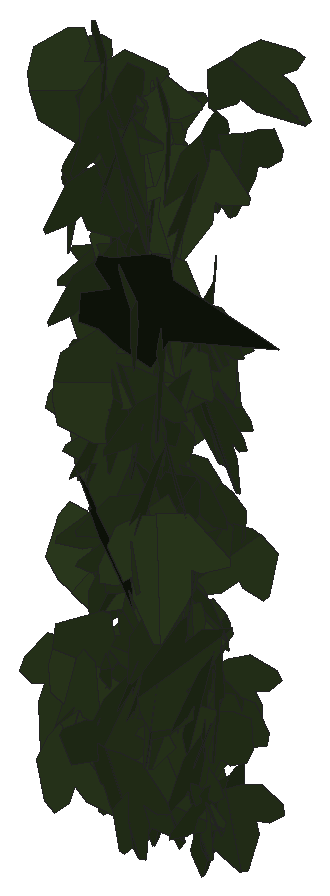
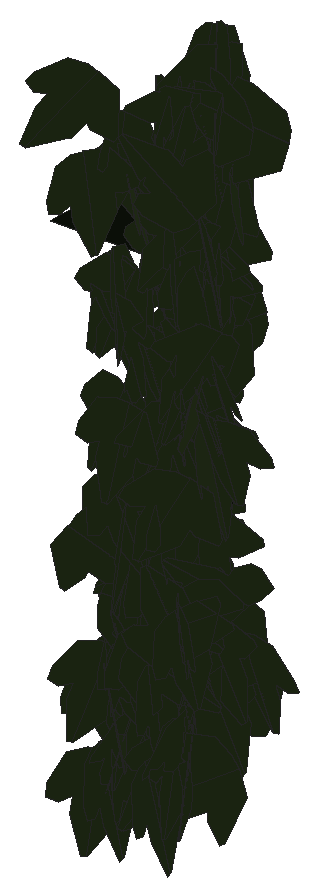
# SketchUp Ruby script. Lengths in inches.
U = 1.inch
M = Sketchup.active_model
def pt(a) = Geom::Point3d.new(a.map { |v| v * U })
def face(e, loops, mat)
  f = e.add_face(loops[0].map { |a| pt(a) })
  loops[1..].each { |l| e.add_face(l.map { |a| pt(a) }).erase! }
  f.material = f.back_material = mat if mat
  f
end
# faces: each face lists its corners as indices into pts; further lists are holes
def faces(e, pts, list, mat = nil) = list.each { |f| face(e, (f[0].is_a?(Array) ? f : [f]).map { |l| l.map { |i| pts[i] } }, mat) }
# xy, xz, yz: faces in a plane at the given z, y or x. An outline is a flat list of corners, or four numbers for a rectangle; further outlines are holes
def ring(l) = l.size == 4 ? [[l[0], l[1]], [l[2], l[1]], [l[2], l[3]], [l[0], l[3]]] : l.each_slice(2).to_a
def flat(e, list, mat, &to3) = list.each { |f| face(e, (f[0].is_a?(Array) ? f : [f]).map { |l| ring(l).map { |u, v| to3.(u, v) } }, mat) }
def xy(e, z, list, mat = nil) = flat(e, list, mat) { |x, y| [x, y, z] }
def xz(e, y, list, mat = nil) = flat(e, list, mat) { |x, z| [x, y, z] }
def yz(e, x, list, mat = nil) = flat(e, list, mat) { |y, z| [x, y, z] }
def lines(e, pts, list) = list.each { |a, b| e.add_line(pt(pts[a]), pt(pts[b])) }
# prism: a flat outline (further loops are holes) pulled along v
def prism(e, loops, v, mat = nil)
  f = face(e, loops, mat); d = Geom::Vector3d.new(v.map { |x| x * U })
  f.pushpull(f.normal.samedirection?(d) ? d.length : -d.length)
end
def box(e, o, s, mat = nil) = prism(e, [[o, [o[0] + s[0], o[1], o[2]], [o[0] + s[0], o[1] + s[1], o[2]], [o[0], o[1] + s[1], o[2]]]], [0, 0, s[2]], mat)
def at(x, y, z, deg = 0) = Geom::Transformation.translation(pt([x, y, z])) * Geom::Transformation.rotation(ORIGIN, Z_AXIS, deg.degrees)
def axes(o, x, y, z) = Geom::Transformation.new([*x, 0, *y, 0, *z, 0, *pt(o).to_a, 1])
def part(name) = M.definitions.add(name)
# library, detail: a bought-in or finely detailed component or shape, given as its bounding box
def library(name, o, s) = part(name).tap { |d| box(d.entities, o, s) }
def detail(e, o, s) = box(e.add_group.entities, o, s)
def put(e, d, t, mat = nil) = e.add_instance(d, t).tap { |i| i.material = mat if mat }
def group(e, t, mat = nil) = e.add_group.tap { |g| g.transformation = t; g.material = mat if mat }.entities
root = M.entities
M.materials.add("efeu1").color = [18, 25, 13]
M.materials.add("efeu2").color = [43, 57, 29]
c1 = part("ivyleaf_10")
p = [[0,0.5,-0.03],[-0.0625,2.02,-0.43],[-0.19,2.01,-0.46],[-0.54,1.05,-0.29],[-0.52,0.625,-0.18],[-0.83,0.76,-0.28],
  [-1.16,0.64,-0.33],[-1.15,0.33,-0.24],[-0.77,-0.39,0.02],[-0.3,-0.51,0.16],[0.04,-0.48,0.23],[-0.02,2.01,-0.4375],
  [-0.06,2.01,-0.43],[0.04,-0.49,0.23],[0.67,-0.49,0.14],[1.38,0.36,-0.2],[1.375,0.51,-0.24],[0.81,0.65,-0.19],
  [0.62,0.59,-0.15],[0.6,1.09,-0.28],[0.5,1.23,-0.31]]
faces(c1.entities,p,[[0,1,2,3,4,5,6,7,8,9,10],[11,12,0,13,14,15,16,17,18,19,20]],"efeu2")
c2 = part("ivyleaf_9")
p = [[1.54,2.16,1.25],[1.36,2.04,1.19],[-0.21,0.99,0.68],[-0.71,1.11,0.82],[-0.85,0.86,0.67],[-0.8,0.17,0.21],
  [-0.9,-0.01,0.1],[-0.67,-0.16,-0.02],[-0.08,-0.08,-0.05],[-0.03,-0.6,-0.4],[0.65,-0.88,-0.66],[0.83,-0.6,-0.49],
  [1.29,-0.42,-0.43],[1.8125,-0.07,-0.26],[1.21,0.44,0.15]]
faces(c2.entities,p,[[0,1,2,3,4,5,6,7,8,9,10,11,12,13,14]],"efeu1")
put(root,c1,axes([509.14,138.66,175.01],[-0.12487,-0.54148,0.08377],[0.01315,-0.08485,-0.57503],[0.59109,-0.1125,0.03049]))
put(root,c1,axes([509.08,137.85,177.79],[0.63301,0.02051,-0.00556],[-0.00502,-0.0199,-0.60959],[-0.02233,0.5858,-0.02052]))
put(root,c1,axes([509.17,137.07,174.02],[0.64268,-0.19201,-0.04798],[-0.04531,0.02022,-0.65026],[0.2084,0.59652,0.0066]))
put(root,c1,axes([508.87,138.21,172.65],[-0.3827,0.09507,-0.52218],[0.51482,-0.09013,-0.39371],[-0.12913,-0.6411,-0.02209]))
put(root,c1,axes([508.7,137.42,182.46],[0.14471,0.01205,-0.68867],[0.68877,-0.00317,0.14467],[-0.00062,-0.7037,-0.01244]))
put(root,c1,axes([509,137.7,175.15],[0.43863,0.21179,-0.47557],[0.31682,0.38486,0.46361],[0.4131,-0.52005,0.14941]))
put(root,c1,axes([509.18,138.58,175.14],[0.39654,-0.42737,0.03226],[0.11124,0.04837,-0.5748],[0.4492,0.36529,0.11386]))
put(root,c1,axes([509.33,138.37,175.4],[-0.35479,-0.44656,0.0359],[0.02472,-0.05949,-0.57386],[0.4831,-0.32492,0.05573]))
put(root,c1,axes([509.38,137.8,180.74],[0.31056,-0.44996,-0.20666],[-0.10102,0.17596,-0.55514],[0.52155,0.30202,0.01553]))
put(root,c1,axes([509.125,137.42,181.51],[0.19807,-0.40948,0.38674],[0.27262,-0.28664,-0.45774],[0.53156,0.29959,0.09065]))
put(root,c1,axes([509.36,138.09,172.95],[0.24083,-0.49273,-0.37457],[-0.01972,0.39561,-0.53309],[0.61862,0.20443,0.12882]))
put(root,c1,axes([509.21,138.66,174.84],[-0.26372,-0.48177,0.15292],[0.07732,0.12856,0.5617],[-0.53849,0.2544,0.00576]))
put(root,c1,axes([509.37,137.71,177.49],[0.1664,-0.66597,-0.03146],[0.00048,0.03254,-0.68639],[0.66671,0.16619,0.00834]))
put(root,c1,axes([509.41,137.53,173.38],[-0.00057,-0.57318,0.15265],[0.00419,-0.14678,-0.59609],[0.63899,0.00045,0.00404]))
put(root,c1,axes([509.5,138.43,175.24],[-0.13521,-0.39389,0.39525],[-0.05313,-0.38018,-0.42665],[0.58874,-0.12477,0.05227]))
put(root,c1,axes([509.72,137.3125,174.05],[-0.47414,-0.04836,0.35073],[-0.35876,-0.06142,-0.45889],[0.08172,-0.55018,0.0204]))
put(root,c1,axes([509.33,137.68,178.71],[0.49544,-0.37884,0.12538],[0.09205,-0.08609,-0.61862],[0.41938,0.46644,-0.01234]))
put(root,c1,axes([509.54,137.85,176.01],[-0.36134,-0.54866,0.07499],[-0.02503,-0.07327,-0.65667],[0.55319,-0.36169,0.01927]))
put(root,c1,axes([509.29,138.56,177.05],[-0.51196,-0.19796,-0.24826],[0.27307,0.00575,-0.52714],[0.19392,-0.53072,0.08689]))
put(root,c1,axes([509.29,137.89,179.07],[0.15858,0.4507,0.35105],[0.06475,0.33434,-0.4914],[-0.60468,0.154,0.03945]))
put(root,c1,axes([509.49,137.35,181.26],[-0.61777,0.06757,-0.01879],[0.02137,0.01354,-0.5988],[-0.07245,-0.57214,-0.01639]))
put(root,c1,axes([509.01,137.65,182.65],[0.00822,0.00838,-0.58657],[0.53618,-0.26787,0.00282],[-0.2892,-0.4964,-0.01143]))
put(root,c1,axes([509.39,138.36,173.36],[-0.08192,0.61733,-0.17364],[0.00439,-0.17451,-0.62249],[-0.64127,-0.08005,0.01792]))
put(root,c1,axes([509.56,137.66,179.85],[-0.08392,-0.55093,0.08387],[-0.02496,-0.07817,-0.57851],[0.60083,-0.0802,-0.01232]))
put(root,c1,axes([509.4375,137.84,178.22],[0.41126,-0.44506,0.10504],[0.06153,-0.08416,-0.60905],[0.48903,0.38487,-0.01171]))
put(root,c1,axes([509.51,138.25,176.6],[-0.11415,-0.55749,-0.10275],[0.06861,0.0882,-0.58824],[0.60761,-0.1147,0.04712]))
put(root,c1,axes([509.52,138.05,177.81],[-0.35046,0.43159,0.164],[0.09673,-0.12993,0.56154],[0.48674,0.33658,0.00649]))
put(root,c1,axes([509.93,138.47,174.19],[-0.19632,-0.05381,0.55093],[-0.51666,-0.22928,-0.19494],[0.25251,-0.51098,0.02946]))
put(root,c1,axes([509.59,137.62,180.05],[-0.36607,-0.45073,-0.01534],[0.01817,0.0058,-0.58642],[0.48671,-0.33922,0.01036]))
put(root,c1,axes([509.55,138.19,172.91],[-0.00889,-0.60241,-0.23675],[0.06063,0.23495,-0.60012],[0.64441,-0.03042,0.0532]))
put(root,c1,axes([509.42,137.49,178.36],[-0.18354,-0.47633,0.33366],[0.10435,0.3061,0.52587],[-0.61141,0.19524,-0.01041]))
put(root,c1,axes([509.53,137.55,178.77],[-0.07467,-0.50124,-0.45425],[0.15323,0.43259,-0.50254],[0.65887,-0.15741,0.06539]))
put(root,c1,axes([509.42,138.08,173.7],[-0.19871,0.24647,0.58049],[0.31709,-0.48706,0.31534],[0.54514,0.37314,0.02818]))
put(root,c1,axes([509.28,138.45,181.63],[-0.3775,-0.1456,0.44551],[0.42649,0.16602,0.39379],[-0.23849,0.52737,-0.00097]))
put(root,c1,axes([509.69,137.65,175.74],[-0.02961,-0.52372,0.22708],[-0.01503,-0.21791,-0.54541],[0.61262,-0.03066,-0.00241]))
put(root,c1,axes([509.76,137.78,177.32],[-0.33227,-0.53823,0.24946],[-0.03247,-0.26899,-0.62363],[0.59234,-0.31666,0.10575]))
put(root,c1,axes([509.72,137.06,183.28],[0.38698,-0.45428,-0.39024],[-0.08482,0.41836,-0.57113],[0.59284,0.35639,0.17301]))
put(root,c1,axes([509.97,137.35,180.0625],[-0.58493,-0.06905,0.27843],[-0.273,-0.11491,-0.56264],[0.12098,-0.59313,0.07659]))
put(root,c1,axes([509.52,136.79,173.09],[0.26424,0.48852,0.38512],[0.09582,0.3663,-0.56352],[-0.65508,0.25063,0.07292]))
put(root,c1,axes([509.8125,138.35,173.78],[0.05243,-0.63569,-0.06027],[0.01195,0.06144,-0.63763],[0.63843,0.05105,0.01688]))
put(root,c1,axes([509.84,136.9375,180.33],[-0.13581,-0.63386,-0.24451],[0.04552,0.2403,-0.64822],[0.67786,-0.14313,-0.00546]))
put(root,c1,axes([509.28,137.1,174.125],[0.10624,0.00216,0.70362],[0.61107,0.35251,-0.09335],[-0.34884,0.61815,0.05077]))
put(root,c1,axes([509.86,138.38,172.22],[0.05985,-0.64034,0.01624],[0.00112,-0.01621,-0.64313],[0.64055,0.05985,-0.00039]))
put(root,c1,axes([509.91,137.85,178.45],[0.34044,-0.44979,-0.21807],[-0.07705,0.20476,-0.56832],[0.53039,0.31844,0.05741]))
put(root,c1,axes([509.95,138.02,175.47],[-0.24327,-0.61296,0.06258],[-0.01611,-0.06093,-0.65943],[0.61594,-0.24369,0.00747]))
put(root,c1,axes([509.9375,137.36,180.33],[-0.62009,0.22343,0.06611],[-0.06123,0.02959,-0.64071],[-0.2433,-0.57691,-0.00726]))
put(root,c1,axes([509.42,137.34,182.14],[-0.13498,-0.00239,0.56842],[0.58728,0.05601,0.12958],[-0.05954,0.55786,-0.01058]))
put(root,c1,axes([509.88,136.85,181.77],[-0.21426,-0.60456,-0.28846],[0.10539,0.26866,-0.64134],[0.66151,-0.23862,0.00874]))
put(root,c1,axes([509.95,137.83,181.61],[0.06508,0.56133,-0.06654],[-0.02303,0.06656,0.58641],[0.60973,-0.0574,0.02925]))
put(root,c1,axes([509.86,137.06,182.98],[0.09541,0.61839,0.18764],[-0.07444,0.19014,-0.64267],[-0.69172,0.06484,0.09504]))
put(root,c1,axes([509.96,137.1875,182.35],[0.35103,-0.55012,-0.08052],[-0.04596,0.06478,-0.66451],[0.59822,0.32778,-0.0038]))
put(root,c1,axes([509.74,137.86,172.46],[-0.34284,-0.36394,-0.40618],[0.33592,0.23705,-0.49593],[0.42964,-0.47575,0.06362]))
put(root,c1,axes([509.99,137.56,176.5],[-0.38172,-0.48256,-0.05548],[0.03984,0.0391,-0.62204],[0.52282,-0.3553,0.0069]))
put(root,c1,axes([509.98,137.66,180.7],[0.15542,-0.63244,-0.21257],[0.00176,0.21865,-0.64923],[0.6672,0.14674,0.05123]))
put(root,c1,axes([509.9,138.13,177.88],[0.01762,0.5546,0.16814],[-0.03797,0.16239,-0.57566],[-0.62274,0.00579,0.03985]))
put(root,c2,axes([509.9,136.74,176.6875],[0.5788,-0.16573,-0.47397],[-0.45392,0.13647,-0.60204],[0.21463,0.73555,0.00491]))
put(root,c1,axes([509.48,137.18,179.55],[0.24218,-0.0734,-0.5652],[0.59158,0.00168,0.23482],[-0.02854,-0.5879,0.07123]))
put(root,c1,axes([509.81,137.64,182.59],[0.45132,0.38393,0.13453],[0.09498,0.09544,-0.59008],[-0.42712,0.42692,0.01093]))
put(root,c1,axes([509.72,137.63,180.625],[0.3125,0.34159,0.37469],[0.24439,0.28042,-0.46552],[-0.47725,0.36727,0.00696]))
put(root,c1,axes([509.8,136.54,178.74],[0.02998,0.12484,0.68277],[0.15502,0.66494,-0.12839],[-0.67656,0.15789,0.00083]))
put(root,c1,axes([510.03,137,178.36],[0.18306,-0.36742,-0.49893],[0.02595,0.50196,-0.39098],[0.6521,0.08317,0.15562]))
put(root,c1,axes([510.09,137.62,174.26],[0.32416,-0.57791,-0.11823],[-0.04442,0.11061,-0.66245],[0.58821,0.32684,0.01513]))
put(root,c1,axes([509.76,137.35,172.74],[-0.42036,-0.04946,-0.40688],[0.42307,0.0147,-0.40724],[0.04896,-0.55167,0.02563]))
put(root,c1,axes([509.98,137.73,178.19],[0.38686,-0.4298,0.14428],[0.10695,-0.09802,-0.58172],[0.47589,0.37141,0.01344]))
put(root,c1,axes([509.96,136.96,173.21],[-0.22323,-0.63266,0.1545],[0.06639,0.14037,0.6707],[-0.64785,0.23238,0.01549]))
put(root,c1,axes([510.35,137.82,171.81],[-0.28384,0.33763,-0.40241],[-0.24179,0.31584,0.44478],[0.49913,0.34501,-0.01337]))
put(root,c1,axes([510.57,137.51,174.22],[-0.22509,0.04974,0.57862],[-0.60309,-0.00413,-0.21717],[-0.01465,-0.59411,0.04995]))
put(root,c1,axes([510.21,137.96,174.11],[-0.31652,-0.58238,-0.04341],[0.01689,0.04023,-0.66282],[0.58375,-0.31694,-0.00436]))
put(root,c1,axes([510.16,136.86,172.93],[-0.68265,0.14988,-0.05558],[0.05249,-0.02659,-0.67542],[-0.16363,-0.63378,0.01519]))
put(root,c1,axes([510.16,136.75,182.96],[0.02044,-0.64359,-0.32281],[0.09461,0.32254,-0.63706],[0.71377,-0.02433,0.09368]))
put(root,c1,axes([510.24,138.61,177.89],[-0.6015,0.07647,0.00593],[-0.00609,0.00085,-0.58466],[-0.08259,-0.55697,-0.00008]))
put(root,c1,axes([510.35,137.61,173.2],[-0.54543,-0.33875,0.10108],[-0.08144,-0.06043,-0.64202],[0.344,-0.55142,0.00827]))
put(root,c1,axes([510.35,137.93,176.91],[-0.65245,0.09455,0.1204],[-0.12192,-0.00217,-0.65898],[-0.09258,-0.66346,0.01931]))
put(root,c1,axes([510.24,137.11,178.66],[-0.63612,0.07548,-0.07644],[0.07782,-0.01597,-0.61753],[-0.08301,-0.59335,0.00689]))
put(root,c1,axes([510.51,138.01,176.29],[-0.45251,-0.25979,0.32296],[-0.23595,-0.23117,-0.50769],[0.36814,-0.46749,0.07158]))
put(root,c1,axes([510.375,137.17,174.73],[0.15623,-0.50167,-0.32406],[-0.09851,0.29798,-0.54298],[0.63016,0.17096,-0.00454]))
put(root,c1,axes([510.25,136.93,182.01],[-0.37119,0.54639,0.0525],[-0.03388,0.0399,-0.67129],[-0.59164,-0.34508,0.00551]))
put(root,c1,axes([510.59,138.4,176.58],[-0.4806,0.03811,0.35329],[-0.36917,-0.05396,-0.45939],[0.00288,-0.55723,0.06864]))
put(root,c1,axes([510.65,138.13,173.88],[-0.48704,-0.08585,0.43355],[-0.42663,-0.07713,-0.49455],[0.1154,-0.64747,0.00143]))
put(root,c1,axes([510.25,136.81,182.69],[-0.29769,0.58841,0.0867],[-0.02488,0.08125,-0.67562],[-0.64135,-0.27627,-0.01403]))
put(root,c1,axes([510.44,138.02,175.16],[-0.6164,0.22371,0.13248],[-0.13594,0.01328,-0.6549],[-0.22163,-0.63034,0.03322]))
put(root,c1,axes([510.37,137.58,182.44],[0.41585,-0.43477,-0.3496],[-0.07351,0.38953,-0.57187],[0.55303,0.3787,0.18687]))
put(root,c1,axes([510.31,138.39,176.125],[0.18244,-0.50568,-0.20922],[0.08997,0.23219,-0.53423],[0.58083,0.12287,0.14847]))
put(root,c1,axes([510.35,137.91,178.85],[0.62158,-0.11678,-0.04123],[-0.04141,0.01042,-0.61075],[0.12659,0.5768,0.00269]))
put(root,c1,axes([510.27,138.02,172.54],[-0.57355,0.20995,-0.23148],[0.19314,-0.14221,-0.60753],[-0.24569,-0.60193,0.0628]))
put(root,c1,axes([509.92,137.91,175.38],[0.28881,0.03466,0.60123],[0.58515,0.14148,-0.28924],[-0.14237,0.65182,0.03081]))
put(root,c1,axes([510.52,137.36,178.33],[-0.11257,-0.67832,-0.10841],[0.02058,0.10648,-0.68759],[0.68662,-0.1144,0.00283]))
put(root,c1,axes([510.625,136.53,180.25],[0.1932,-0.12301,-0.65014],[-0.17228,0.61998,-0.17435],[0.66617,0.19601,0.14346]))
put(root,c1,axes([510.39,137.63,180.07],[-0.54085,0.22627,-0.2532],[0.12957,-0.28753,-0.53455],[-0.33476,-0.47685,0.20218]))
put(root,c1,axes([510.51,137.2,177.45],[0.32159,-0.59057,-0.01523],[-0.00126,0.01666,-0.67241],[0.59076,0.32152,0.00686]))
put(root,c1,axes([510.59,137.58,176.41],[-0.02318,-0.57546,0.00235],[-0.00033,-0.00225,-0.59889],[0.6215,-0.02147,-0.00023]))
put(root,c1,axes([510.5,137.61,177.55],[-0.34296,0.57727,-0.03177],[0.01692,-0.0269,-0.67146],[-0.5779,-0.34338,-0.0008]))
put(root,c1,axes([510.5,137.28,176.43],[0.00037,0.65266,0.11754],[-0.02407,0.11748,-0.65222],[-0.66272,-0.0039,0.02376]))
put(root,c1,axes([510.55,137.91,181.3125],[0.27872,-0.53105,0.07811],[0.06338,-0.05489,-0.61334],[0.57577,0.26312,0.0297]))
put(root,c1,axes([510.63,137.77,175.68],[0.43174,-0.46357,-0.22263],[-0.06067,0.24274,-0.6231],[0.51067,0.42076,0.11419]))
put(root,c1,axes([510.49,137.91,181.62],[0.58611,0.25182,0.00176],[0.00651,-0.00899,-0.62211],[-0.2719,0.54263,-0.01112]))
put(root,c1,axes([510.66,137.74,174.1],[0.12704,0.5378,-0.2886],[-0.19889,-0.23748,-0.55983],[-0.62259,0.1856,0.11995]))
put(root,c1,axes([510.43,137.2,172.53],[-0.22429,-0.34357,-0.52427],[0.3394,0.39618,-0.41545],[0.56471,-0.37456,0.04146]))
put(root,c1,axes([510.71,138.22,173.42],[0.24535,-0.48522,-0.18064],[-0.08142,0.15649,-0.5572],[0.55062,0.23935,-0.00191]))
put(root,c1,axes([510.59,138.11,172.79],[-0.13571,0.55127,0.05979],[-0.01133,0.05657,-0.58802],[-0.59849,-0.12607,-0.00242]))
put(root,c1,axes([510.8,138.09,173.51],[-0.56933,-0.31366,0.12038],[-0.07724,-0.10832,-0.64754],[0.32697,-0.57174,0.05664]))
put(root,c1,axes([510.75,138.73,181.69],[-0.2931,-0.4834,0.0378],[-0.01199,-0.03545,-0.57649],[0.5234,-0.27151,0.00797]))
put(root,c1,axes([510.76,138.27,172.15],[0.03634,-0.66389,0.00621],[0.00139,-0.00614,-0.66488],[0.66392,0.03635,0.00106]))
put(root,c1,axes([510.96,138.49,175.8],[0.22681,0.31096,-0.42742],[-0.44452,-0.16588,-0.34926],[-0.33496,0.43069,0.17408]))
put(root,c1,axes([510.48,137.64,176.57],[-0.52234,0.03072,0.36251],[0.36887,-0.08785,0.50091],[0.08217,0.58966,0.05574]))
put(root,c1,axes([510.69,137.96,182],[0.01524,-0.56508,-0.21951],[0.10192,0.21059,-0.5798],[0.64345,-0.01997,0.09704]))
put(root,c1,axes([510.66,138.25,177.91],[-0.5074,0.28958,-0.10187],[0.08559,-0.05808,-0.5739],[-0.31886,-0.47639,0.00805]))
put(root,c1,axes([510.76,137.82,173.87],[-0.05804,-0.60108,-0.09138],[0.06956,0.08207,-0.62488],[0.65237,-0.06223,0.0585]))
put(root,c1,axes([510.49,137.37,179.26],[0.32167,-0.35586,0.42914],[0.35307,-0.25951,-0.47816],[0.4708,0.43776,0.06539]))
put(root,c1,axes([510.69,137.0625,175.35],[-0.05386,-0.47309,-0.48273],[0.16928,0.45938,-0.4691],[0.65436,-0.15779,0.08162]))
put(root,c1,axes([510.5,137.27,174.33],[0.34417,-0.2834,0.44751],[0.32809,-0.3053,-0.4431],[0.44945,0.43989,-0.01923]))
put(root,c1,axes([510.8,137.98,179.81],[0.2124,-0.53587,-0.20525],[-0.00925,0.20594,-0.59043],[0.61667,0.18766,0.06183]))
put(root,c1,axes([510.92,137.85,173.37],[-0.35566,-0.50179,0.23544],[-0.07816,-0.23154,-0.61156],[0.54874,-0.35821,0.06549]))
put(root,c1,axes([510.77,138.05,174.6875],[-0.03261,-0.28697,0.49385],[0.09892,-0.47161,-0.29035],[0.59099,0.0631,0.07585]))
put(root,c1,axes([510.73,138.39,173.82],[-0.43284,-0.34097,-0.2019],[0.17581,0.108,-0.54677],[0.38556,-0.43202,0.02266]))
put(root,c1,axes([510.84,137.74,173.11],[0.10673,-0.59206,-0.3014],[0.01151,0.30687,-0.59873],[0.66427,0.08981,0.05881]))
put(root,c1,axes([510.86,137.98,179.17],[0.58252,-0.2182,-0.15893],[-0.14295,0.07996,-0.6046],[0.24967,0.55487,0.02463]))
put(root,c1,axes([510.89,138.3,172.05],[-0.47025,-0.36663,-0.07146],[0.05591,0.0452,-0.59198],[0.39896,-0.43848,-0.00127]))
put(root,c1,axes([510.8125,137.82,179.53],[-0.57045,0.2272,-0.09254],[0.08909,-0.03342,-0.59798],[-0.24801,-0.5346,-0.00195]))
put(root,c1,axes([510.75,136.94,176.53],[0.50264,0.45989,0.02463],[0.0183,0.01655,-0.68046],[-0.497,0.46571,-0.00015]))
put(root,c1,axes([510.82,137.82,179.48],[-0.5797,0.10337,-0.20572],[0.20184,-0.07345,-0.56735],[-0.13176,-0.56731,0.03597]))
put(root,c2,axes([510.36,136.62,180.3],[0.18457,0.22644,-0.71654],[0.4925,0.52083,0.29145],[0.56758,-0.52557,-0.01989]))
put(root,c1,axes([510.75,138.0625,174.25],[0.51649,-0.34605,0.23266],[0.24496,-0.04793,-0.61509],[0.33745,0.56444,0.09041]))
put(root,c1,axes([511.05,137.56,174.375],[0.23799,-0.6195,-0.05972],[-0.01351,0.05878,-0.66359],[0.62223,0.23822,0.00843]))
put(root,c1,axes([511.09,136.625,174.6],[0.10375,-0.12143,0.71883],[-0.15711,0.70528,0.14182],[-0.71188,-0.17335,0.07346]))
put(root,c1,axes([510.88,138.65,182.96],[-0.39864,-0.22644,-0.36903],[0.33996,0.16484,-0.44994],[0.30182,-0.48475,0.01938]))
